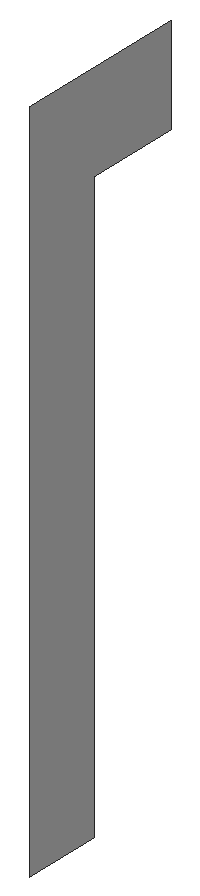
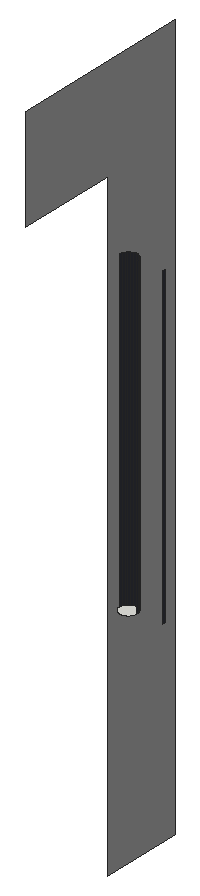
# SketchUp Ruby script. Lengths in inches.
U = 1.inch
M = Sketchup.active_model
def pt(a) = Geom::Point3d.new(a.map { |v| v * U })
def face(e, loops, mat)
  f = e.add_face(loops[0].map { |a| pt(a) })
  loops[1..].each { |l| e.add_face(l.map { |a| pt(a) }).erase! }
  f.material = f.back_material = mat if mat
  f
end
# faces: each face lists its corners as indices into pts; further lists are holes
def faces(e, pts, list, mat = nil) = list.each { |f| face(e, (f[0].is_a?(Array) ? f : [f]).map { |l| l.map { |i| pts[i] } }, mat) }
# xy, xz, yz: faces in a plane at the given z, y or x. An outline is a flat list of corners, or four numbers for a rectangle; further outlines are holes
def ring(l) = l.size == 4 ? [[l[0], l[1]], [l[2], l[1]], [l[2], l[3]], [l[0], l[3]]] : l.each_slice(2).to_a
def flat(e, list, mat, &to3) = list.each { |f| face(e, (f[0].is_a?(Array) ? f : [f]).map { |l| ring(l).map { |u, v| to3.(u, v) } }, mat) }
def xy(e, z, list, mat = nil) = flat(e, list, mat) { |x, y| [x, y, z] }
def xz(e, y, list, mat = nil) = flat(e, list, mat) { |x, z| [x, y, z] }
def yz(e, x, list, mat = nil) = flat(e, list, mat) { |y, z| [x, y, z] }
def lines(e, pts, list) = list.each { |a, b| e.add_line(pt(pts[a]), pt(pts[b])) }
# prism: a flat outline (further loops are holes) pulled along v
def prism(e, loops, v, mat = nil)
  f = face(e, loops, mat); d = Geom::Vector3d.new(v.map { |x| x * U })
  f.pushpull(f.normal.samedirection?(d) ? d.length : -d.length)
end
def box(e, o, s, mat = nil) = prism(e, [[o, [o[0] + s[0], o[1], o[2]], [o[0] + s[0], o[1] + s[1], o[2]], [o[0], o[1] + s[1], o[2]]]], [0, 0, s[2]], mat)
def at(x, y, z, deg = 0) = Geom::Transformation.translation(pt([x, y, z])) * Geom::Transformation.rotation(ORIGIN, Z_AXIS, deg.degrees)
def axes(o, x, y, z) = Geom::Transformation.new([*x, 0, *y, 0, *z, 0, *pt(o).to_a, 1])
def part(name) = M.definitions.add(name)
# library, detail: a bought-in or finely detailed component or shape, given as its bounding box
def library(name, o, s) = part(name).tap { |d| box(d.entities, o, s) }
def detail(e, o, s) = box(e.add_group.entities, o, s)
def put(e, d, t, mat = nil) = e.add_instance(d, t).tap { |i| i.material = mat if mat }
def group(e, t, mat = nil) = e.add_group.tap { |g| g.transformation = t; g.material = mat if mat }.entities
root = M.entities
M.materials.add("[Blinds Vertical Stripe Gray]").color = [160, 160, 160]
M.materials.add("[Formica Laminate Dark]").color = [50, 53, 60]
xy(root,22.1875,[[187.96,106,187.78,106.02,187.61,106.09,187.47,106.2,187.36,106.34,187.29,106.51,187.27,106.6875,187.29,106.87,187.36,107.03,187.47,107.17,187.61,107.28,187.78,107.35,187.96,107.375,188.14,107.35,188.3,107.28,188.44,107.17,188.55,107.03,188.62,106.87,188.65,106.6875,188.62,106.51,188.55,106.34,188.44,106.2,188.3,106.09,188.14,106.02]])
yz(root,192.64,[[96.24,0,96.24,57.8125,111,57.8125,111,49.625,102.91,49.625,102.91,0]],"[Blinds Vertical Stripe Gray]")
p = [[187.61,106.09,22.1875],[187.78,106.02,22.1875],[187.78,106.02,47.21],[187.61,106.09,47.21],[187.96,106,22.1875],[187.96,106,47.21],
  [188.14,106.02,22.1875],[188.14,106.02,47.21],[188.3,106.09,22.1875],[188.3,106.09,47.21],[187.47,106.2,22.1875],[187.47,106.2,47.21],
  [188.44,106.2,22.1875],[188.44,106.2,47.21],[187.36,106.34,22.1875],[187.36,106.34,47.21],[188.55,106.34,22.1875],[188.55,106.34,47.21],
  [187.29,106.51,22.1875],[187.29,106.51,47.21],[188.62,106.51,22.1875],[188.62,106.51,47.21],[185.18,106.51,22.1875],[185.21,106.6875,22.1875],
  [185.21,106.6875,47.21],[185.18,106.51,47.21],[187.27,106.6875,22.1875],[187.27,106.6875,47.21],[188.65,106.6875,22.1875],[188.65,106.6875,47.21]]
faces(root,p,[[0,1,2,3],[1,4,5,2],[4,6,7,5],[6,8,9,7],[10,0,3,11],[8,12,13,9],[14,10,11,15],[12,16,17,13],
  [18,14,15,19],[16,20,21,17],[22,23,24,25],[26,18,19,27],[20,28,29,21]],"[Formica Laminate Dark]")
